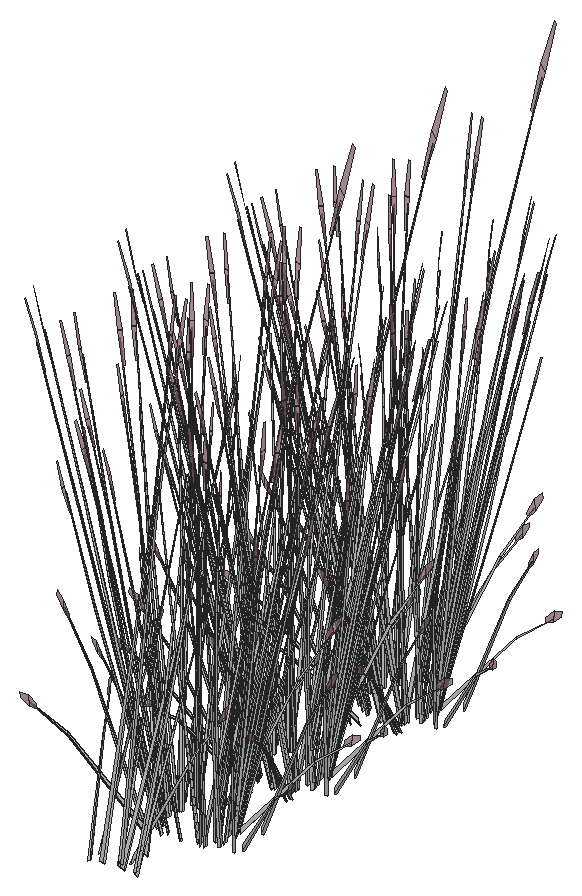
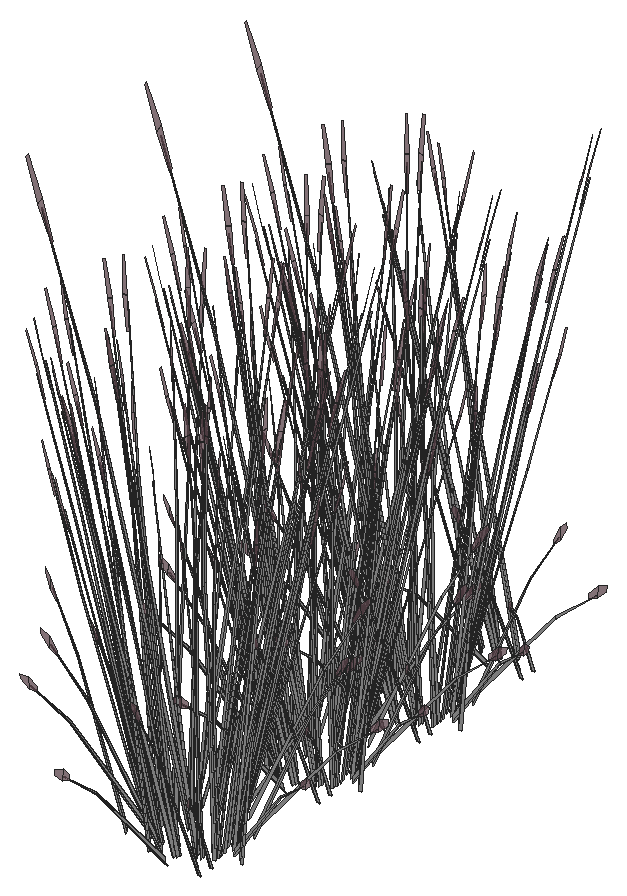
# SketchUp Ruby script. Lengths in inches.
U = 1.inch
M = Sketchup.active_model
def pt(a) = Geom::Point3d.new(a.map { |v| v * U })
def face(e, loops, mat)
  f = e.add_face(loops[0].map { |a| pt(a) })
  loops[1..].each { |l| e.add_face(l.map { |a| pt(a) }).erase! }
  f.material = f.back_material = mat if mat
  f
end
# faces: each face lists its corners as indices into pts; further lists are holes
def faces(e, pts, list, mat = nil) = list.each { |f| face(e, (f[0].is_a?(Array) ? f : [f]).map { |l| l.map { |i| pts[i] } }, mat) }
# xy, xz, yz: faces in a plane at the given z, y or x. An outline is a flat list of corners, or four numbers for a rectangle; further outlines are holes
def ring(l) = l.size == 4 ? [[l[0], l[1]], [l[2], l[1]], [l[2], l[3]], [l[0], l[3]]] : l.each_slice(2).to_a
def flat(e, list, mat, &to3) = list.each { |f| face(e, (f[0].is_a?(Array) ? f : [f]).map { |l| ring(l).map { |u, v| to3.(u, v) } }, mat) }
def xy(e, z, list, mat = nil) = flat(e, list, mat) { |x, y| [x, y, z] }
def xz(e, y, list, mat = nil) = flat(e, list, mat) { |x, z| [x, y, z] }
def yz(e, x, list, mat = nil) = flat(e, list, mat) { |y, z| [x, y, z] }
def lines(e, pts, list) = list.each { |a, b| e.add_line(pt(pts[a]), pt(pts[b])) }
# prism: a flat outline (further loops are holes) pulled along v
def prism(e, loops, v, mat = nil)
  f = face(e, loops, mat); d = Geom::Vector3d.new(v.map { |x| x * U })
  f.pushpull(f.normal.samedirection?(d) ? d.length : -d.length)
end
def box(e, o, s, mat = nil) = prism(e, [[o, [o[0] + s[0], o[1], o[2]], [o[0] + s[0], o[1] + s[1], o[2]], [o[0], o[1] + s[1], o[2]]]], [0, 0, s[2]], mat)
def at(x, y, z, deg = 0) = Geom::Transformation.translation(pt([x, y, z])) * Geom::Transformation.rotation(ORIGIN, Z_AXIS, deg.degrees)
def axes(o, x, y, z) = Geom::Transformation.new([*x, 0, *y, 0, *z, 0, *pt(o).to_a, 1])
def part(name) = M.definitions.add(name)
# library, detail: a bought-in or finely detailed component or shape, given as its bounding box
def library(name, o, s) = part(name).tap { |d| box(d.entities, o, s) }
def detail(e, o, s) = box(e.add_group.entities, o, s)
def put(e, d, t, mat = nil) = e.add_instance(d, t).tap { |i| i.material = mat if mat }
def group(e, t, mat = nil) = e.add_group.tap { |g| g.transformation = t; g.material = mat if mat }.entities
root = M.entities
M.materials.add("LightPink_Translucent").color = [144, 107, 117]
M.materials["LightPink_Translucent"].alpha = 0.75
M.materials.add("[_0053_Ivory_]").color = [200, 200, 200]
c1 = part("blade")
p = [[2.15,0.21,22],[0,0.17,0],[0.09,0.45,0],[2.18,0.31,22],[2.29,0.31,22],[0.38,0.45,0],
  [2.48,0.24,33],[2.49,0.24,33],[2.48,0.22,33]]
faces(c1.entities,p,[[0,1,2,3],[4,5,2,3],[6,3,4,7],[8,0,3,6]])
c2 = part("seeds")
p = [[0.3,-0.1,1.38],[-0.01,-0.03,1.59],[-0.01,-0.03,0.03],[0.14,-0.07,-0.07],[0.29,-0.03,3],[0.15,0.01,3.11]]
faces(c2.entities,p,[[0,1,2,3],[1,0,4,5]],"LightPink_Translucent")
c3 = part("blade with seeds")
put(c3.entities,c1,at(0,0,0))
put(c3.entities,c2,axes([2.4,0.25,30.99],[1.5799,-0.05474,1.17369],[-0.12525,1.92788,0.29478],[-0.07173,-0.02425,1.56792]))
put(root,c3,axes([632.31,312.61,256.7],[-0.1831,0.48359,0.35414],[-0.53419,-0.14105,-0.4572],[-0.04898,-0.1947,0.87481]),"[_0053_Ivory_]")
put(root,c3,axes([633.68,312.82,256.39],[0.43249,0.42907,0.48003],[-0.45929,0.37004,0.3958],[0.07978,-0.2013,0.9933]),"[_0053_Ivory_]")
put(root,c3,axes([631.07,312.19,257.08],[-0.40534,0.60286,-0.13619],[-0.58702,-0.34732,-0.75594],[-0.20405,-0.17032,1.14864]),"[_0053_Ivory_]")
put(root,c3,axes([633.84,312.86,256.38],[0.49911,0.0293,0.0643],[-0.01368,0.44245,0.50621],[0.05223,-0.16948,0.77189]),"[_0053_Ivory_]")
put(root,c3,axes([633.46,313.16,256.7],[-0.41095,0.33109,0.35414],[-0.38901,-0.37805,-0.4572],[0.05919,-0.19208,0.87481]),"[_0053_Ivory_]")
put(root,c3,axes([632.71,307.27,256.38],[-0.27604,0.39948,0.0643],[-0.39309,-0.23258,0.50621],[0.12709,0.12808,0.77189]),"[_0053_Ivory_]")
put(root,c3,axes([632.06,308.61,257.3],[0.4197,-0.36076,-0.06488],[0.38456,0.39511,-0.29416],[0.02707,0.11196,0.97024]),"[_0053_Ivory_]")
put(root,c3,axes([632.82,307.16,256.39],[-0.60408,0.14432,0.48003],[-0.10484,-0.56611,0.3958],[0.14207,0.16684,0.9933]),"[_0053_Ivory_]")
put(root,c3,axes([629.51,312.02,256.37],[-0.13068,-0.00444,1.74944],[-0.41604,0.44388,-0.27667],[-0.22198,-0.0907,0.14031]),"[_0053_Ivory_]")
put(root,c3,axes([634.45,314.23,256.6875],[-0.56181,-0.34675,-0.1216],[0.32367,-0.50216,-0.67495],[0.15873,-0.17455,1.02557]),"[_0053_Ivory_]")
put(root,c3,axes([631.18,307.33,256.38],[-0.44753,0.21372,0.0643],[-0.21905,-0.38973,0.50621],[0.04322,0.1718,0.77189]),"[_0053_Ivory_]")
put(root,c3,axes([628.56,306.72,256.37],[-0.0151,0.12444,1.74944],[0.42844,0.43292,-0.27667],[-0.11216,0.20472,0.14031]),"[_0053_Ivory_]")
put(root,c3,axes([629.93,306.44,257.05],[0.6675,0.03116,-0.13498],[-0.01824,0.58993,-0.74919],[-0.04637,0.2272,1.13838]),"[_0053_Ivory_]")
put(root,c3,axes([631.16,307.09,256.6875],[0.59433,-0.29278,-0.1216],[0.29207,0.51964,-0.67495],[0.07842,0.21898,1.02557]),"[_0053_Ivory_]")
put(root,c3,axes([631.33,307.29,256.72],[-0.59846,-0.1644,0.53283],[0.20464,-0.54049,0.43934],[0.03596,0.21255,1.10256]),"[_0053_Ivory_]")
put(root,c3,axes([631.03,312.69,256.7],[0.0938,0.50652,0.35414],[-0.53623,0.13375,-0.4572],[-0.14403,-0.14515,0.87481]),"[_0053_Ivory_]")
put(root,c3,axes([629.42,313.02,256.75],[0.50157,-0.46409,0.53763],[0.43258,0.49285,0.4433],[-0.23532,-0.08561,1.11249]),"[_0053_Ivory_]")
put(root,c3,axes([635.83,314.08,256.36],[-0.07933,-0.00478,1.77383],[-0.32942,-0.51175,-0.16761],[0.13229,-0.16826,0.31391]),"[_0053_Ivory_]")
put(root,c3,axes([629.65,313.02,256.38],[0.03058,-0.47819,0.0643],[0.4618,0.01311,0.50621],[-0.1769,-0.05004,0.77189]),"[_0053_Ivory_]")
put(root,c3,axes([634.18,314.18,256.7],[-0.52868,0.08987,0.35414],[-0.1396,-0.51376,-0.4572],[0.1515,-0.13799,0.87481]),"[_0053_Ivory_]")
put(root,c3,axes([628.51,307.99,256.36],[0.0689,-0.03797,1.77383],[0.5695,0.25254,-0.16761],[-0.01338,0.21027,0.31391]),"[_0053_Ivory_]")
put(root,c3,axes([634.66,314.1,256.38],[0.41695,0.26447,0.0643],[-0.24275,0.37662,0.50621],[0.13368,-0.12176,0.77189]),"[_0053_Ivory_]")
put(root,c3,axes([634.54,313.99,256.39],[0.15063,0.57876,0.48003],[-0.59087,0.10045,0.3958],[0.17414,-0.13612,0.9933]),"[_0053_Ivory_]")
put(root,c3,axes([636.13,314.69,256.37],[0.08428,-0.09579,1.74944],[-0.10787,-0.58756,-0.27667],[0.21147,-0.1114,0.14031]),"[_0053_Ivory_]")
put(root,c3,axes([631.02,308.26,256.37],[0.07699,0.10127,1.74944],[0.6213,0.03978,-0.27667],[0.06248,0.22333,0.14031]),"[_0053_Ivory_]")
put(root,c3,axes([629.01,312.4,256.36],[0.04503,0.06276,1.77383],[-0.21706,0.56413,-0.16761],[-0.21983,0.00408,0.31391]),"[_0053_Ivory_]")
put(root,c3,axes([629.96,313.38,256.7],[0.34557,0.39372,0.35414],[-0.39459,0.37271,-0.4572],[-0.20048,-0.05671,0.87481]),"[_0053_Ivory_]")
put(root,c3,axes([629.87,313.13,256.6875],[-0.03252,0.63953,-0.1216],[-0.61574,-0.01748,-0.67495],[-0.23714,-0.04442,1.02557]),"[_0053_Ivory_]")
put(root,c3,axes([634.47,315.58,256.6875],[-0.30559,-0.56943,-0.1216],[0.54237,-0.27983,-0.67495],[0.22856,-0.07513,1.02557]),"[_0053_Ivory_]")
put(root,c3,axes([634.26,315.41,256.7],[-0.50475,-0.17543,0.35414],[0.14722,-0.5118,-0.4572],[0.20322,-0.04693,0.87481]),"[_0053_Ivory_]")
put(root,c3,axes([628.98,314.48,256.39],[0.17159,-0.57338,0.48003],[0.56413,0.19607,0.3958],[-0.22185,0.03446,0.9933]),"[_0053_Ivory_]")
put(root,c3,axes([628.93,314.32,256.38],[-0.22307,-0.42878,0.0643],[0.40677,-0.20987,0.50621],[-0.17931,0.04141,0.77189]),"[_0053_Ivory_]")
put(root,c3,axes([634.72,315.57,256.38],[0.22307,0.42878,0.0643],[-0.40677,0.20987,0.50621],[0.17931,-0.04141,0.77189]),"[_0053_Ivory_]")
put(root,c3,axes([634.68,315.42,256.39],[-0.17159,0.57338,0.48003],[-0.56413,-0.19607,0.3958],[0.22185,-0.03446,0.9933]),"[_0053_Ivory_]")
put(root,c3,axes([629.39,314.48,256.7],[0.50475,0.17543,0.35414],[-0.14722,0.5118,-0.4572],[-0.20322,0.04693,0.87481]),"[_0053_Ivory_]")
put(root,c3,axes([635.6875,317.27,256.36],[-0.05492,-0.05505,1.77383],[0.12013,-0.59013,-0.16761],[0.21632,-0.0377,0.31391]),"[_0053_Ivory_]")
put(root,c3,axes([628.54,314.88,256.37],[-0.09918,0.08165,1.74944],[0.00844,0.59653,-0.27667],[-0.22734,0.07758,0.14031]),"[_0053_Ivory_]")
put(root,c3,axes([629.18,314.3125,256.6875],[0.30559,0.56943,-0.1216],[-0.54237,0.27983,-0.67495],[-0.22856,0.07513,1.02557]),"[_0053_Ivory_]")
put(root,c3,axes([633.79,316.77,256.6875],[0.03252,-0.63953,-0.1216],[0.61574,0.01748,-0.67495],[0.23714,0.04442,1.02557]),"[_0053_Ivory_]")
put(root,c3,axes([633.69,316.52,256.7],[-0.34557,-0.39372,0.35414],[0.39459,-0.37271,-0.4572],[0.20048,0.05671,0.87481]),"[_0053_Ivory_]")
put(root,c3,axes([631.55,321.16,256.37],[-0.0929,-0.08817,1.74944],[-0.61994,0.0559,-0.27667],[-0.09894,-0.21089,0.14031]),"[_0053_Ivory_]")
put(root,c3,axes([634.32,316.38,256.37],[0.13029,-0.01064,1.74944],[0.35737,-0.48855,-0.27667],[0.23175,0.06449,0.14031]),"[_0053_Ivory_]")
put(root,c3,axes([629.11,315.9,256.39],[-0.15063,-0.57876,0.48003],[0.59087,-0.10045,0.3958],[-0.17414,0.13612,0.9933]),"[_0053_Ivory_]")
put(root,c3,axes([629,315.79,256.38],[-0.41695,-0.26447,0.0643],[0.24275,-0.37662,0.50621],[-0.13368,0.12176,0.77189]),"[_0053_Ivory_]")
put(root,c3,axes([634.33,322.24,256.37],[-0.00586,-0.12516,1.74944],[-0.49517,-0.36172,-0.27667],[0.07656,-0.21927,0.14031]),"[_0053_Ivory_]")
put(root,c3,axes([634.2,321.79,256.36],[-0.06168,0.04803,1.77383],[-0.60432,-0.16205,-0.16761],[-0.02188,-0.20961,0.31391]),"[_0053_Ivory_]")
put(root,c3,axes([629.48,315.71,256.7],[0.52868,-0.08987,0.35414],[0.1396,0.51376,-0.4572],[-0.1515,0.13799,0.87481]),"[_0053_Ivory_]")
put(root,c3,axes([627.4375,315.48,256.36],[0.07751,0.01687,1.77383],[0.23978,0.55562,-0.16761],[-0.15867,0.14583,0.31391]),"[_0053_Ivory_]")
put(root,c3,axes([634.01,316.87,256.38],[-0.03058,0.47819,0.0643],[-0.4618,-0.01311,0.50621],[0.1769,0.05004,0.77189]),"[_0053_Ivory_]")
put(root,c3,axes([630.91,320.87,256.36],[-0.01133,0.07538,1.77383],[-0.55883,0.27355,-0.16761],[-0.16445,-0.13983,0.31391]),"[_0053_Ivory_]")
put(root,c3,axes([634.05,316.72,256.39],[-0.44783,0.41436,0.48003],[-0.38623,-0.44004,0.3958],[0.21011,0.07643,0.9933]),"[_0053_Ivory_]")
put(root,c3,axes([630.79,322.2,256.75],[0.67657,-0.16163,0.53763],[0.11742,0.63404,0.4433],[-0.15912,-0.18687,1.11249]),"[_0053_Ivory_]")
put(root,c3,axes([632.32,322.32,256.39],[0.59846,0.1644,0.48003],[-0.20464,0.54049,0.3958],[-0.03596,-0.21255,0.9933]),"[_0053_Ivory_]")
put(root,c3,axes([632.49,322.52,256.6875],[-0.59433,0.29278,-0.1216],[-0.29207,-0.51964,-0.67495],[-0.07842,-0.21898,1.02557]),"[_0053_Ivory_]")
put(root,c3,axes([633.72,323.17,256.6875],[-0.6675,-0.03116,-0.1216],[0.01824,-0.58993,-0.67495],[0.04637,-0.2272,1.02557]),"[_0053_Ivory_]")
put(root,c3,axes([628.28,317.17,257.3],[0.53595,0.16786,-0.06488],[-0.16486,0.51664,-0.29416],[-0.08766,0.07844,0.97024]),"[_0053_Ivory_]")
put(root,c3,axes([632.48,322.28,256.38],[0.44753,-0.21372,0.0643],[0.21905,0.38973,0.50621],[-0.04322,-0.1718,0.77189]),"[_0053_Ivory_]")
put(root,c3,axes([632.625,317.2,256.7],[-0.0938,-0.50652,0.35414],[0.53623,-0.13375,-0.4572],[0.14403,0.14515,0.87481]),"[_0053_Ivory_]")
put(root,c3,axes([632.98,314.29,256.13],[-0.52482,-0.32674,1.38283],[0.55416,-0.50872,0.59665],[0.16933,0.30658,1.33663]),"[_0053_Ivory_]")
put(root,c3,axes([629.2,315.66,256.6875],[0.56181,0.34675,-0.1216],[-0.32367,0.50216,-0.67495],[-0.15873,0.17455,1.02557]),"[_0053_Ivory_]")
put(root,c3,axes([630.94,322.34,256.38],[0.27604,-0.39948,0.0643],[0.39309,0.23258,0.50621],[-0.12709,-0.12808,0.77189]),"[_0053_Ivory_]")
put(root,c3,axes([632.57,317.46,256.6875],[0.36191,-0.53827,-0.1216],[0.52412,0.3101,-0.67495],[0.18219,0.15207,1.02557]),"[_0053_Ivory_]")
put(root,c3,axes([630.1875,316.74,256.7],[0.41095,-0.33109,0.35414],[0.38901,0.37805,-0.4572],[-0.05919,0.19208,0.87481]),"[_0053_Ivory_]")
put(root,c3,axes([632.31,322.72,256.7],[-0.1831,0.48359,0.35414],[-0.53419,-0.14105,-0.4572],[-0.04898,-0.1947,0.87481]),"[_0053_Ivory_]")
put(root,c3,axes([632.1,317.91,256.36],[0.0018,-0.07613,1.77383],[0.52048,-0.3359,-0.16761],[0.18079,0.11989,0.31391]),"[_0053_Ivory_]")
put(root,c3,axes([629.82,317.04,256.38],[-0.49911,-0.0293,0.0643],[0.01368,-0.44245,0.50621],[-0.05223,0.16948,0.77189]),"[_0053_Ivory_]")
put(root,c3,axes([633.68,322.92,256.39],[0.43249,0.42907,0.48003],[-0.45929,0.37004,0.3958],[0.07978,-0.2013,0.9933]),"[_0053_Ivory_]")
put(root,c3,axes([631.07,322.3,257.08],[-0.40534,0.60286,-0.13619],[-0.58702,-0.34732,-0.75594],[-0.20405,-0.17032,1.14864]),"[_0053_Ivory_]")
put(root,c3,axes([629.98,317.08,256.39],[-0.43249,-0.42907,0.48003],[0.45929,-0.37004,0.3958],[-0.07978,0.2013,0.9933]),"[_0053_Ivory_]")
put(root,c3,axes([633.84,322.96,256.38],[0.49911,0.0293,0.0643],[-0.01368,0.44245,0.50621],[0.05223,-0.16948,0.77189]),"[_0053_Ivory_]")
put(root,c3,axes([631.34,317.28,256.7],[0.1831,-0.48359,0.35414],[0.53419,0.14105,-0.4572],[0.04898,0.1947,0.87481]),"[_0053_Ivory_]")
put(root,c3,axes([633.46,323.26,256.7],[-0.41095,0.33109,0.35414],[-0.38901,-0.37805,-0.4572],[0.05919,-0.19208,0.87481]),"[_0053_Ivory_]")
put(root,c3,axes([632.71,317.66,256.38],[-0.27604,0.39948,0.0643],[-0.39309,-0.23258,0.50621],[0.12709,0.12808,0.77189]),"[_0053_Ivory_]")
put(root,c3,axes([629.51,322.125,256.37],[-0.13068,-0.00444,1.74944],[-0.41604,0.44388,-0.27667],[-0.22198,-0.0907,0.14031]),"[_0053_Ivory_]")
put(root,c3,axes([634.45,324.34,256.6875],[-0.56181,-0.34675,-0.1216],[0.32367,-0.50216,-0.67495],[0.15873,-0.17455,1.02557]),"[_0053_Ivory_]")
put(root,c3,axes([632.06,319,257.3],[0.4197,-0.36076,-0.06488],[0.38456,0.39511,-0.29416],[0.02707,0.11196,0.97024]),"[_0053_Ivory_]")
put(root,c3,axes([632.82,317.55,256.39],[-0.60408,0.14432,0.48003],[-0.10484,-0.56611,0.3958],[0.14207,0.16684,0.9933]),"[_0053_Ivory_]")
put(root,c3,axes([631.03,322.8,256.7],[0.0938,0.50652,0.35414],[-0.53623,0.13375,-0.4572],[-0.14403,-0.14515,0.87481]),"[_0053_Ivory_]")
put(root,c3,axes([629.42,323.13,256.75],[0.50157,-0.46409,0.53763],[0.43258,0.49285,0.4433],[-0.23532,-0.08561,1.11249]),"[_0053_Ivory_]")
put(root,c3,axes([635.83,324.19,256.36],[-0.07933,-0.00478,1.77383],[-0.32942,-0.51175,-0.16761],[0.13229,-0.16826,0.31391]),"[_0053_Ivory_]")
put(root,c3,axes([631.18,317.72,256.38],[-0.44753,0.21372,0.0643],[-0.21905,-0.38973,0.50621],[0.04322,0.1718,0.77189]),"[_0053_Ivory_]")
put(root,c3,axes([628.56,317.11,256.37],[-0.0151,0.12444,1.74944],[0.42844,0.43292,-0.27667],[-0.11216,0.20472,0.14031]),"[_0053_Ivory_]")
put(root,c3,axes([629.93,316.83,257.05],[0.6675,0.03116,-0.13498],[-0.01824,0.58993,-0.74919],[-0.04637,0.2272,1.13838]),"[_0053_Ivory_]")
put(root,c3,axes([631.16,317.48,256.6875],[0.59433,-0.29278,-0.1216],[0.29207,0.51964,-0.67495],[0.07842,0.21898,1.02557]),"[_0053_Ivory_]")
put(root,c3,axes([631.33,317.68,256.72],[-0.59846,-0.1644,0.53283],[0.20464,-0.54049,0.43934],[0.03596,0.21255,1.10256]),"[_0053_Ivory_]")
put(root,c3,axes([629.65,323.13,256.38],[0.03058,-0.47819,0.0643],[0.4618,0.01311,0.50621],[-0.1769,-0.05004,0.77189]),"[_0053_Ivory_]")
put(root,c3,axes([634.18,324.29,256.7],[-0.52868,0.08987,0.35414],[-0.1396,-0.51376,-0.4572],[0.1515,-0.13799,0.87481]),"[_0053_Ivory_]")
put(root,c3,axes([628.51,318.38,256.36],[0.0689,-0.03797,1.77383],[0.5695,0.25254,-0.16761],[-0.01338,0.21027,0.31391]),"[_0053_Ivory_]")
put(root,c3,axes([634.66,324.21,256.38],[0.41695,0.26447,0.0643],[-0.24275,0.37662,0.50621],[0.13368,-0.12176,0.77189]),"[_0053_Ivory_]")
put(root,c3,axes([634.54,324.1,256.39],[0.15063,0.57876,0.48003],[-0.59087,0.10045,0.3958],[0.17414,-0.13612,0.9933]),"[_0053_Ivory_]")
put(root,c3,axes([636.13,324.8,256.37],[0.08428,-0.09579,1.74944],[-0.10787,-0.58756,-0.27667],[0.21147,-0.1114,0.14031]),"[_0053_Ivory_]")
put(root,c3,axes([629.01,322.5,256.36],[0.04503,0.06276,1.77383],[-0.21706,0.56413,-0.16761],[-0.21983,0.00408,0.31391]),"[_0053_Ivory_]")
put(root,c3,axes([631.02,318.65,256.37],[0.07699,0.10127,1.74944],[0.6213,0.03978,-0.27667],[0.06248,0.22333,0.14031]),"[_0053_Ivory_]")
put(root,c3,axes([629.96,323.48,256.7],[0.34557,0.39372,0.35414],[-0.39459,0.37271,-0.4572],[-0.20048,-0.05671,0.87481]),"[_0053_Ivory_]")
put(root,c3,axes([629.87,323.23,256.6875],[-0.03252,0.63953,-0.1216],[-0.61574,-0.01748,-0.67495],[-0.23714,-0.04442,1.02557]),"[_0053_Ivory_]")
put(root,c3,axes([634.47,325.6875,256.6875],[-0.30559,-0.56943,-0.1216],[0.54237,-0.27983,-0.67495],[0.22856,-0.07513,1.02557]),"[_0053_Ivory_]")
put(root,c3,axes([634.26,325.52,256.7],[-0.50475,-0.17543,0.35414],[0.14722,-0.5118,-0.4572],[0.20322,-0.04693,0.87481]),"[_0053_Ivory_]")
put(root,c3,axes([628.98,324.58,256.39],[0.17159,-0.57338,0.48003],[0.56413,0.19607,0.3958],[-0.22185,0.03446,0.9933]),"[_0053_Ivory_]")
put(root,c3,axes([628.93,324.43,256.38],[-0.22307,-0.42878,0.0643],[0.40677,-0.20987,0.50621],[-0.17931,0.04141,0.77189]),"[_0053_Ivory_]")
put(root,c3,axes([634.72,325.68,256.38],[0.22307,0.42878,0.0643],[-0.40677,0.20987,0.50621],[0.17931,-0.04141,0.77189]),"[_0053_Ivory_]")
put(root,c3,axes([634.68,325.52,256.39],[-0.17159,0.57338,0.48003],[-0.56413,-0.19607,0.3958],[0.22185,-0.03446,0.9933]),"[_0053_Ivory_]")
put(root,c3,axes([629.39,324.59,256.7],[0.50475,0.17543,0.35414],[-0.14722,0.5118,-0.4572],[-0.20322,0.04693,0.87481]),"[_0053_Ivory_]")
put(root,c3,axes([635.6875,327.38,256.36],[-0.05492,-0.05505,1.77383],[0.12013,-0.59013,-0.16761],[0.21632,-0.0377,0.31391]),"[_0053_Ivory_]")
put(root,c3,axes([628.54,324.99,256.37],[-0.09918,0.08165,1.74944],[0.00844,0.59653,-0.27667],[-0.22734,0.07758,0.14031]),"[_0053_Ivory_]")
put(root,c3,axes([629.18,324.42,256.6875],[0.30559,0.56943,-0.1216],[-0.54237,0.27983,-0.67495],[-0.22856,0.07513,1.02557]),"[_0053_Ivory_]")
put(root,c3,axes([633.79,326.87,256.6875],[0.03252,-0.63953,-0.1216],[0.61574,0.01748,-0.67495],[0.23714,0.04442,1.02557]),"[_0053_Ivory_]")
put(root,c3,axes([633.69,326.62,256.7],[-0.34557,-0.39372,0.35414],[0.39459,-0.37271,-0.4572],[0.20048,0.05671,0.87481]),"[_0053_Ivory_]")
put(root,c3,axes([634.32,326.49,256.37],[0.13029,-0.01064,1.74944],[0.35737,-0.48855,-0.27667],[0.23175,0.06449,0.14031]),"[_0053_Ivory_]")
put(root,c3,axes([629.11,326.01,256.39],[-0.15063,-0.57876,0.48003],[0.59087,-0.10045,0.3958],[-0.17414,0.13612,0.9933]),"[_0053_Ivory_]")
put(root,c3,axes([629,325.9,256.38],[-0.41695,-0.26447,0.0643],[0.24275,-0.37662,0.50621],[-0.13368,0.12176,0.77189]),"[_0053_Ivory_]")
put(root,c3,axes([629.48,325.82,256.7],[0.52868,-0.08987,0.35414],[0.1396,0.51376,-0.4572],[-0.1515,0.13799,0.87481]),"[_0053_Ivory_]")
put(root,c3,axes([627.4375,325.59,256.36],[0.07751,0.01687,1.77383],[0.23978,0.55562,-0.16761],[-0.15867,0.14583,0.31391]),"[_0053_Ivory_]")
put(root,c3,axes([634.01,326.98,256.38],[-0.03058,0.47819,0.0643],[-0.4618,-0.01311,0.50621],[0.1769,0.05004,0.77189]),"[_0053_Ivory_]")
put(root,c3,axes([634.05,326.83,256.39],[-0.44783,0.41436,0.48003],[-0.38623,-0.44004,0.3958],[0.21011,0.07643,0.9933]),"[_0053_Ivory_]")
put(root,c3,axes([628.28,327.28,257.3],[0.53595,0.16786,-0.06488],[-0.16486,0.51664,-0.29416],[-0.08766,0.07844,0.97024]),"[_0053_Ivory_]")
put(root,c3,axes([632.625,327.31,256.7],[-0.0938,-0.50652,0.35414],[0.53623,-0.13375,-0.4572],[0.14403,0.14515,0.87481]),"[_0053_Ivory_]")
put(root,c3,axes([631.55,333.11,256.37],[-0.0929,-0.08817,1.74944],[-0.61994,0.0559,-0.27667],[-0.09894,-0.21089,0.14031]),"[_0053_Ivory_]")
put(root,c3,axes([632.98,324.39,256.13],[-0.52482,-0.32674,1.38283],[0.55416,-0.50872,0.59665],[0.16933,0.30658,1.33663]),"[_0053_Ivory_]")
put(root,c3,axes([629.2,325.77,256.6875],[0.56181,0.34675,-0.1216],[-0.32367,0.50216,-0.67495],[-0.15873,0.17455,1.02557]),"[_0053_Ivory_]")
put(root,c3,axes([632.57,327.57,256.6875],[0.36191,-0.53827,-0.1216],[0.52412,0.3101,-0.67495],[0.18219,0.15207,1.02557]),"[_0053_Ivory_]")
put(root,c3,axes([630.1875,326.84,256.7],[0.41095,-0.33109,0.35414],[0.38901,0.37805,-0.4572],[-0.05919,0.19208,0.87481]),"[_0053_Ivory_]")
put(root,c3,axes([634.33,334.2,256.37],[-0.00586,-0.12516,1.74944],[-0.49517,-0.36172,-0.27667],[0.07656,-0.21927,0.14031]),"[_0053_Ivory_]")
put(root,c3,axes([634.2,333.75,256.36],[-0.06168,0.04803,1.77383],[-0.60432,-0.16205,-0.16761],[-0.02188,-0.20961,0.31391]),"[_0053_Ivory_]")
put(root,c3,axes([632.1,328.01,256.36],[0.0018,-0.07613,1.77383],[0.52048,-0.3359,-0.16761],[0.18079,0.11989,0.31391]),"[_0053_Ivory_]")
put(root,c3,axes([629.82,327.14,256.38],[-0.49911,-0.0293,0.0643],[0.01368,-0.44245,0.50621],[-0.05223,0.16948,0.77189]),"[_0053_Ivory_]")
put(root,c3,axes([629.98,327.18,256.39],[-0.43249,-0.42907,0.48003],[0.45929,-0.37004,0.3958],[-0.07978,0.2013,0.9933]),"[_0053_Ivory_]")
put(root,c3,axes([631.34,327.39,256.7],[0.1831,-0.48359,0.35414],[0.53419,0.14105,-0.4572],[0.04898,0.1947,0.87481]),"[_0053_Ivory_]")
put(root,c3,axes([630.91,332.83,256.36],[-0.01133,0.07538,1.77383],[-0.55883,0.27355,-0.16761],[-0.16445,-0.13983,0.31391]),"[_0053_Ivory_]")
put(root,c3,axes([632.71,327.76,256.38],[-0.27604,0.39948,0.0643],[-0.39309,-0.23258,0.50621],[0.12709,0.12808,0.77189]),"[_0053_Ivory_]")
put(root,c3,axes([630.79,334.16,256.75],[0.67657,-0.16163,0.53763],[0.11742,0.63404,0.4433],[-0.15912,-0.18687,1.11249]),"[_0053_Ivory_]")
put(root,c3,axes([632.06,329.11,257.3],[0.4197,-0.36076,-0.06488],[0.38456,0.39511,-0.29416],[0.02707,0.11196,0.97024]),"[_0053_Ivory_]")
put(root,c3,axes([632.82,327.65,256.39],[-0.60408,0.14432,0.48003],[-0.10484,-0.56611,0.3958],[0.14207,0.16684,0.9933]),"[_0053_Ivory_]")
put(root,c3,axes([632.32,334.28,256.39],[0.59846,0.1644,0.48003],[-0.20464,0.54049,0.3958],[-0.03596,-0.21255,0.9933]),"[_0053_Ivory_]")
put(root,c3,axes([632.49,334.48,256.6875],[-0.59433,0.29278,-0.1216],[-0.29207,-0.51964,-0.67495],[-0.07842,-0.21898,1.02557]),"[_0053_Ivory_]")
put(root,c3,axes([633.72,335.13,256.6875],[-0.6675,-0.03116,-0.1216],[0.01824,-0.58993,-0.67495],[0.04637,-0.2272,1.02557]),"[_0053_Ivory_]")
put(root,c3,axes([632.48,334.24,256.38],[0.44753,-0.21372,0.0643],[0.21905,0.38973,0.50621],[-0.04322,-0.1718,0.77189]),"[_0053_Ivory_]")
put(root,c3,axes([631.18,327.82,256.38],[-0.44753,0.21372,0.0643],[-0.21905,-0.38973,0.50621],[0.04322,0.1718,0.77189]),"[_0053_Ivory_]")
put(root,c3,axes([628.56,327.21,256.37],[-0.0151,0.12444,1.74944],[0.42844,0.43292,-0.27667],[-0.11216,0.20472,0.14031]),"[_0053_Ivory_]")
put(root,c3,axes([629.93,326.93,257.05],[0.6675,0.03116,-0.13498],[-0.01824,0.58993,-0.74919],[-0.04637,0.2272,1.13838]),"[_0053_Ivory_]")
put(root,c3,axes([631.16,327.59,256.6875],[0.59433,-0.29278,-0.1216],[0.29207,0.51964,-0.67495],[0.07842,0.21898,1.02557]),"[_0053_Ivory_]")
put(root,c3,axes([631.33,327.78,256.72],[-0.59846,-0.1644,0.53283],[0.20464,-0.54049,0.43934],[0.03596,0.21255,1.10256]),"[_0053_Ivory_]")
put(root,c3,axes([630.94,334.3,256.38],[0.27604,-0.39948,0.0643],[0.39309,0.23258,0.50621],[-0.12709,-0.12808,0.77189]),"[_0053_Ivory_]")
put(root,c3,axes([632.31,334.68,256.7],[-0.1831,0.48359,0.35414],[-0.53419,-0.14105,-0.4572],[-0.04898,-0.1947,0.87481]),"[_0053_Ivory_]")
put(root,c3,axes([633.68,334.88,256.39],[0.43249,0.42907,0.48003],[-0.45929,0.37004,0.3958],[0.07978,-0.2013,0.9933]),"[_0053_Ivory_]")
put(root,c3,axes([631.07,334.26,257.08],[-0.40534,0.60286,-0.13619],[-0.58702,-0.34732,-0.75594],[-0.20405,-0.17032,1.14864]),"[_0053_Ivory_]")
put(root,c3,axes([633.84,334.92,256.38],[0.49911,0.0293,0.0643],[-0.01368,0.44245,0.50621],[0.05223,-0.16948,0.77189]),"[_0053_Ivory_]")
put(root,c3,axes([633.46,335.22,256.7],[-0.41095,0.33109,0.35414],[-0.38901,-0.37805,-0.4572],[0.05919,-0.19208,0.87481]),"[_0053_Ivory_]")
put(root,c3,axes([628.51,328.49,256.36],[0.0689,-0.03797,1.77383],[0.5695,0.25254,-0.16761],[-0.01338,0.21027,0.31391]),"[_0053_Ivory_]")
put(root,c3,axes([629.51,334.09,256.37],[-0.13068,-0.00444,1.74944],[-0.41604,0.44388,-0.27667],[-0.22198,-0.0907,0.14031]),"[_0053_Ivory_]")
put(root,c3,axes([634.45,336.29,256.6875],[-0.56181,-0.34675,-0.1216],[0.32367,-0.50216,-0.67495],[0.15873,-0.17455,1.02557]),"[_0053_Ivory_]")
put(root,c3,axes([631.03,334.76,256.7],[0.0938,0.50652,0.35414],[-0.53623,0.13375,-0.4572],[-0.14403,-0.14515,0.87481]),"[_0053_Ivory_]")
put(root,c3,axes([631.02,328.75,256.37],[0.07699,0.10127,1.74944],[0.6213,0.03978,-0.27667],[0.06248,0.22333,0.14031]),"[_0053_Ivory_]")
put(root,c3,axes([629.42,335.09,256.75],[0.50157,-0.46409,0.53763],[0.43258,0.49285,0.4433],[-0.23532,-0.08561,1.11249]),"[_0053_Ivory_]")
put(root,c3,axes([635.83,336.14,256.36],[-0.07933,-0.00478,1.77383],[-0.32942,-0.51175,-0.16761],[0.13229,-0.16826,0.31391]),"[_0053_Ivory_]")
put(root,c3,axes([629.65,335.09,256.38],[0.03058,-0.47819,0.0643],[0.4618,0.01311,0.50621],[-0.1769,-0.05004,0.77189]),"[_0053_Ivory_]")
put(root,c3,axes([634.18,336.25,256.7],[-0.52868,0.08987,0.35414],[-0.1396,-0.51376,-0.4572],[0.1515,-0.13799,0.87481]),"[_0053_Ivory_]")
put(root,c3,axes([634.66,336.17,256.38],[0.41695,0.26447,0.0643],[-0.24275,0.37662,0.50621],[0.13368,-0.12176,0.77189]),"[_0053_Ivory_]")
put(root,c3,axes([634.54,336.05,256.39],[0.15063,0.57876,0.48003],[-0.59087,0.10045,0.3958],[0.17414,-0.13612,0.9933]),"[_0053_Ivory_]")
put(root,c3,axes([636.13,336.75,256.37],[0.08428,-0.09579,1.74944],[-0.10787,-0.58756,-0.27667],[0.21147,-0.1114,0.14031]),"[_0053_Ivory_]")
put(root,c3,axes([629.01,334.46,256.36],[0.04503,0.06276,1.77383],[-0.21706,0.56413,-0.16761],[-0.21983,0.00408,0.31391]),"[_0053_Ivory_]")
put(root,c3,axes([629.96,335.44,256.7],[0.34557,0.39372,0.35414],[-0.39459,0.37271,-0.4572],[-0.20048,-0.05671,0.87481]),"[_0053_Ivory_]")
put(root,c3,axes([629.87,335.19,256.6875],[-0.03252,0.63953,-0.1216],[-0.61574,-0.01748,-0.67495],[-0.23714,-0.04442,1.02557]),"[_0053_Ivory_]")
put(root,c3,axes([634.47,337.65,256.6875],[-0.30559,-0.56943,-0.1216],[0.54237,-0.27983,-0.67495],[0.22856,-0.07513,1.02557]),"[_0053_Ivory_]")
put(root,c3,axes([634.26,337.48,256.7],[-0.50475,-0.17543,0.35414],[0.14722,-0.5118,-0.4572],[0.20322,-0.04693,0.87481]),"[_0053_Ivory_]")
put(root,c3,axes([628.98,336.54,256.39],[0.17159,-0.57338,0.48003],[0.56413,0.19607,0.3958],[-0.22185,0.03446,0.9933]),"[_0053_Ivory_]")
put(root,c3,axes([628.93,336.39,256.38],[-0.22307,-0.42878,0.0643],[0.40677,-0.20987,0.50621],[-0.17931,0.04141,0.77189]),"[_0053_Ivory_]")
put(root,c3,axes([634.72,337.63,256.38],[0.22307,0.42878,0.0643],[-0.40677,0.20987,0.50621],[0.17931,-0.04141,0.77189]),"[_0053_Ivory_]")
put(root,c3,axes([634.68,337.48,256.39],[-0.17159,0.57338,0.48003],[-0.56413,-0.19607,0.3958],[0.22185,-0.03446,0.9933]),"[_0053_Ivory_]")
put(root,c3,axes([629.39,336.55,256.7],[0.50475,0.17543,0.35414],[-0.14722,0.5118,-0.4572],[-0.20322,0.04693,0.87481]),"[_0053_Ivory_]")
put(root,c3,axes([635.6875,339.34,256.36],[-0.05492,-0.05505,1.77383],[0.12013,-0.59013,-0.16761],[0.21632,-0.0377,0.31391]),"[_0053_Ivory_]")
put(root,c3,axes([628.54,336.94,256.37],[-0.09918,0.08165,1.74944],[0.00844,0.59653,-0.27667],[-0.22734,0.07758,0.14031]),"[_0053_Ivory_]")
put(root,c3,axes([629.18,336.375,256.6875],[0.30559,0.56943,-0.1216],[-0.54237,0.27983,-0.67495],[-0.22856,0.07513,1.02557]),"[_0053_Ivory_]")
put(root,c3,axes([633.79,338.83,256.6875],[0.03252,-0.63953,-0.1216],[0.61574,0.01748,-0.67495],[0.23714,0.04442,1.02557]),"[_0053_Ivory_]")
put(root,c3,axes([633.69,338.58,256.7],[-0.34557,-0.39372,0.35414],[0.39459,-0.37271,-0.4572],[0.20048,0.05671,0.87481]),"[_0053_Ivory_]")
put(root,c3,axes([634.32,338.45,256.37],[0.13029,-0.01064,1.74944],[0.35737,-0.48855,-0.27667],[0.23175,0.06449,0.14031]),"[_0053_Ivory_]")
put(root,c3,axes([629.11,337.97,256.39],[-0.15063,-0.57876,0.48003],[0.59087,-0.10045,0.3958],[-0.17414,0.13612,0.9933]),"[_0053_Ivory_]")
put(root,c3,axes([629,337.86,256.38],[-0.41695,-0.26447,0.0643],[0.24275,-0.37662,0.50621],[-0.13368,0.12176,0.77189]),"[_0053_Ivory_]")
put(root,c3,axes([629.48,337.78,256.7],[0.52868,-0.08987,0.35414],[0.1396,0.51376,-0.4572],[-0.1515,0.13799,0.87481]),"[_0053_Ivory_]")
put(root,c3,axes([627.4375,337.55,256.36],[0.07751,0.01687,1.77383],[0.23978,0.55562,-0.16761],[-0.15867,0.14583,0.31391]),"[_0053_Ivory_]")
put(root,c3,axes([634.01,338.9375,256.38],[-0.03058,0.47819,0.0643],[-0.4618,-0.01311,0.50621],[0.1769,0.05004,0.77189]),"[_0053_Ivory_]")
put(root,c3,axes([634.05,338.78,256.39],[-0.44783,0.41436,0.48003],[-0.38623,-0.44004,0.3958],[0.21011,0.07643,0.9933]),"[_0053_Ivory_]")
put(root,c3,axes([628.28,339.23,257.3],[0.53595,0.16786,-0.06488],[-0.16486,0.51664,-0.29416],[-0.08766,0.07844,0.97024]),"[_0053_Ivory_]")
put(root,c3,axes([632.625,339.26,256.7],[-0.0938,-0.50652,0.35414],[0.53623,-0.13375,-0.4572],[0.14403,0.14515,0.87481]),"[_0053_Ivory_]")
put(root,c3,axes([632.98,336.35,256.13],[-0.52482,-0.32674,1.38283],[0.55416,-0.50872,0.59665],[0.16933,0.30658,1.33663]),"[_0053_Ivory_]")
put(root,c3,axes([629.2,337.73,256.6875],[0.56181,0.34675,-0.1216],[-0.32367,0.50216,-0.67495],[-0.15873,0.17455,1.02557]),"[_0053_Ivory_]")
put(root,c3,axes([632.57,339.53,256.6875],[0.36191,-0.53827,-0.1216],[0.52412,0.3101,-0.67495],[0.18219,0.15207,1.02557]),"[_0053_Ivory_]")
put(root,c3,axes([630.1875,338.8,256.7],[0.41095,-0.33109,0.35414],[0.38901,0.37805,-0.4572],[-0.05919,0.19208,0.87481]),"[_0053_Ivory_]")
put(root,c3,axes([632.1,339.97,256.36],[0.0018,-0.07613,1.77383],[0.52048,-0.3359,-0.16761],[0.18079,0.11989,0.31391]),"[_0053_Ivory_]")
put(root,c3,axes([629.82,339.1,256.38],[-0.49911,-0.0293,0.0643],[0.01368,-0.44245,0.50621],[-0.05223,0.16948,0.77189]),"[_0053_Ivory_]")
put(root,c3,axes([629.98,339.14,256.39],[-0.43249,-0.42907,0.48003],[0.45929,-0.37004,0.3958],[-0.07978,0.2013,0.9933]),"[_0053_Ivory_]")
put(root,c3,axes([631.34,339.34,256.7],[0.1831,-0.48359,0.35414],[0.53419,0.14105,-0.4572],[0.04898,0.1947,0.87481]),"[_0053_Ivory_]")
put(root,c3,axes([632.71,339.72,256.38],[-0.27604,0.39948,0.0643],[-0.39309,-0.23258,0.50621],[0.12709,0.12808,0.77189]),"[_0053_Ivory_]")
put(root,c3,axes([632.06,341.07,257.3],[0.4197,-0.36076,-0.06488],[0.38456,0.39511,-0.29416],[0.02707,0.11196,0.97024]),"[_0053_Ivory_]")
put(root,c3,axes([632.82,339.61,256.39],[-0.60408,0.14432,0.48003],[-0.10484,-0.56611,0.3958],[0.14207,0.16684,0.9933]),"[_0053_Ivory_]")
put(root,c3,axes([631.18,339.78,256.38],[-0.44753,0.21372,0.0643],[-0.21905,-0.38973,0.50621],[0.04322,0.1718,0.77189]),"[_0053_Ivory_]")
put(root,c3,axes([628.56,339.17,256.37],[-0.0151,0.12444,1.74944],[0.42844,0.43292,-0.27667],[-0.11216,0.20472,0.14031]),"[_0053_Ivory_]")
put(root,c3,axes([629.93,338.89,257.05],[0.6675,0.03116,-0.13498],[-0.01824,0.58993,-0.74919],[-0.04637,0.2272,1.13838]),"[_0053_Ivory_]")
put(root,c3,axes([631.16,339.55,256.6875],[0.59433,-0.29278,-0.1216],[0.29207,0.51964,-0.67495],[0.07842,0.21898,1.02557]),"[_0053_Ivory_]")
put(root,c3,axes([631.33,339.74,256.72],[-0.59846,-0.1644,0.53283],[0.20464,-0.54049,0.43934],[0.03596,0.21255,1.10256]),"[_0053_Ivory_]")
put(root,c3,axes([628.51,340.45,256.36],[0.0689,-0.03797,1.77383],[0.5695,0.25254,-0.16761],[-0.01338,0.21027,0.31391]),"[_0053_Ivory_]")
put(root,c3,axes([631.02,340.71,256.37],[0.07699,0.10127,1.74944],[0.6213,0.03978,-0.27667],[0.06248,0.22333,0.14031]),"[_0053_Ivory_]")
